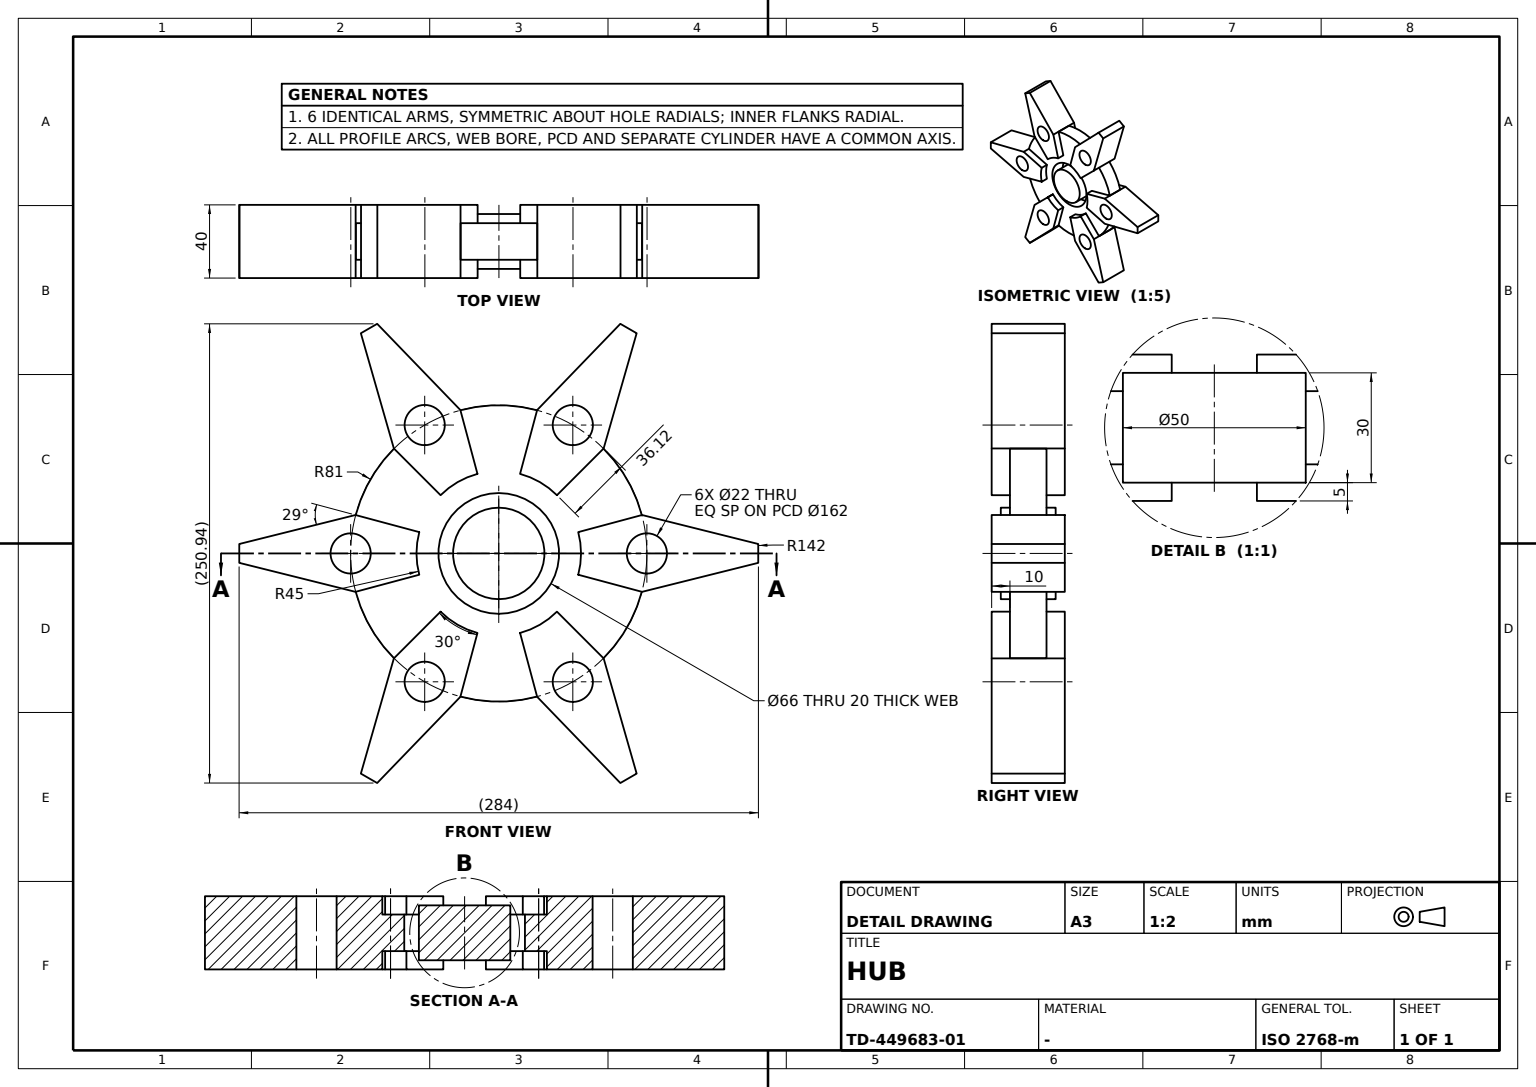
solid
v1 (125.470546,-66.49167,-20)
v2 (125.470546,-66.49167,20)
e1 v1 v2 LINE
v3 (120.318748,-75.414845,20)
e2 v3 v2 CIRCLE(AX(P(0,0,20),D(0,0,1),D(1,0,0)),142)
v4 (120.318748,-75.414845,-20)
e3 v4 v3 LINE
e4 v4 v1 CIRCLE(AX(P(0,0,-20),D(0,0,1),D(1,0,0)),142)
face CYL(AX(P(0,0,0),D(0,0,1),D(0,1,0)),142) [e1 -e2 -e3 e4]
v5 (11.646857,43.466662,20)
v6 (-11.646857,43.466662,20)
e5 v5 v6 CIRCLE(AX(P(0,0,20),D(0,0,1),D(1,0,0)),45)
v7 (-11.646857,43.466662,10)
e6 v7 v6 LINE
v8 (11.646857,43.466662,10)
e7 v8 v7 CIRCLE(AX(P(0,0,10),D(0,0,1),D(1,0,0)),45)
e8 v8 v5 LINE
face CYL(AX(P(0,0,0),D(0,0,1),D(0,1,0)),45) rev [e5 -e6 -e7 e8]
v9 (-31.819805,31.819805,-20)
v10 (-43.466662,11.646857,-20)
e9 v9 v10 CIRCLE(AX(P(0,0,-20),D(0,0,1),D(1,0,0)),45)
v11 (-31.819805,31.819805,-10)
e10 v9 v11 LINE
v12 (-43.466662,11.646857,-10)
e11 v11 v12 CIRCLE(AX(P(0,0,-10),D(0,0,1),D(1,0,0)),45)
e12 v10 v12 LINE
face CYL(AX(P(0,0,0),D(0,0,1),D(0,1,0)),45) rev [-e9 e10 e11 -e12]
v13 (-59.148058,-40.5,-20)
e13 v13 v13 CIRCLE(AX(P(-70.148058,-40.5,-20),D(0,0,1),D(1,0,0)),11)
v14 (-59.148058,-40.5,20)
e14 v14 v14 CIRCLE(AX(P(-70.148058,-40.5,20),D(0,0,1),D(1,0,0)),11)
face CYL(AX(P(-70.148058,-40.5,0),D(0,0,1),D(0,1,0)),11) rev [-e13] [e14]
v15 (-11.646857,-43.466662,20)
v16 (11.646857,-43.466662,20)
e15 v15 v16 CIRCLE(AX(P(0,0,20),D(0,0,1),D(1,0,0)),45)
v17 (11.646857,-43.466662,10)
e16 v17 v16 LINE
v18 (-11.646857,-43.466662,10)
e17 v18 v17 CIRCLE(AX(P(0,0,10),D(0,0,1),D(1,0,0)),45)
e18 v18 v15 LINE
face CYL(AX(P(0,0,0),D(0,0,1),D(0,1,0)),45) rev [e15 -e16 -e17 e18]
v19 (33,0,10)
e19 v19 v19 CIRCLE(AX(P(0,0,10),D(0,0,1),D(1,0,0)),33)
v20 (-20.964343,78.239992,10)
e20 v7 v20 LINE
v21 (-57.275649,57.275649,10)
e21 v20 v21 CIRCLE(AX(P(0,0,10),D(0,0,1),D(1,0,0)),81)
v22 (-31.819805,31.819805,10)
e22 v22 v21 LINE
v23 (-43.466662,11.646857,10)
e23 v22 v23 CIRCLE(AX(P(0,0,10),D(0,0,1),D(1,0,0)),45)
v24 (-78.239992,20.964343,10)
e24 v23 v24 LINE
v25 (-78.239992,-20.964343,10)
e25 v24 v25 CIRCLE(AX(P(0,0,10),D(0,0,1),D(1,0,0)),81)
v26 (-43.466662,-11.646857,10)
e26 v26 v25 LINE
v27 (-31.819805,-31.819805,10)
e27 v26 v27 CIRCLE(AX(P(0,0,10),D(0,0,1),D(1,0,0)),45)
v28 (-57.275649,-57.275649,10)
e28 v27 v28 LINE
v29 (-20.964343,-78.239992,10)
e29 v28 v29 CIRCLE(AX(P(0,0,10),D(0,0,1),D(1,0,0)),81)
e30 v29 v18 LINE
v30 (20.964343,-78.239992,10)
e31 v30 v17 LINE
v31 (57.275649,-57.275649,10)
e32 v30 v31 CIRCLE(AX(P(0,0,10),D(0,0,1),D(1,0,0)),81)
v32 (31.819805,-31.819805,10)
e33 v31 v32 LINE
v33 (43.466662,-11.646857,10)
e34 v32 v33 CIRCLE(AX(P(0,0,10),D(0,0,1),D(1,0,0)),45)
v34 (78.239992,-20.964343,10)
e35 v34 v33 LINE
v35 (78.239992,20.964343,10)
e36 v34 v35 CIRCLE(AX(P(0,0,10),D(0,0,1),D(1,0,0)),81)
v36 (43.466662,11.646857,10)
e37 v35 v36 LINE
v37 (31.819805,31.819805,10)
e38 v36 v37 CIRCLE(AX(P(0,0,10),D(0,0,1),D(1,0,0)),45)
v38 (57.275649,57.275649,10)
e39 v38 v37 LINE
v39 (20.964343,78.239992,10)
e40 v38 v39 CIRCLE(AX(P(0,0,10),D(0,0,1),D(1,0,0)),81)
e41 v8 v39 LINE
face PLANE(AX(P(0,0,10),D(0,0,1),D(0,1,0))) [-e19] [e20 e21 -e22 e23 e24 e25 -e26 e27 e28 e29 e30 e17 -e31 e32 e33 e34 -e35 e36 e37 e38 -e39 e40 -e41 e7]
v40 (-57.275649,-57.275649,-10)
e42 v40 v28 LINE
v41 (-31.819805,-31.819805,20)
e43 v27 v41 LINE
v42 (-57.362403,-57.362403,20)
e44 v41 v42 LINE
v43 (-57.362403,-57.362403,-20)
e45 v43 v42 LINE
v44 (-31.819805,-31.819805,-20)
e46 v44 v43 LINE
v45 (-31.819805,-31.819805,-10)
e47 v44 v45 LINE
e48 v45 v40 LINE
face PLANE(AX(P(-31.819805,-31.819805,0),D(-0.707106781,0.707106781,0),D(-0.707106781,-0.707106781,0))) rev [e42 -e28 e43 e44 -e45 -e46 e47 e48]
v46 (-11.646857,-43.466662,-20)
v47 (-11.646857,-43.466662,-10)
e49 v46 v47 LINE
v48 (11.646857,-43.466662,-10)
e50 v47 v48 CIRCLE(AX(P(0,0,-10),D(0,0,1),D(1,0,0)),45)
v49 (11.646857,-43.466662,-20)
e51 v49 v48 LINE
e52 v46 v49 CIRCLE(AX(P(0,0,-20),D(0,0,1),D(1,0,0)),45)
face CYL(AX(P(0,0,0),D(0,0,1),D(0,1,0)),45) rev [e49 e50 -e51 -e52]
v50 (-57.275649,57.275649,-10)
e53 v11 v50 LINE
v51 (-57.362403,57.362403,-20)
e54 v9 v51 LINE
v52 (-57.362403,57.362403,20)
e55 v51 v52 LINE
v53 (-31.819805,31.819805,20)
e56 v53 v52 LINE
e57 v22 v53 LINE
e58 v50 v21 LINE
face PLANE(AX(P(-31.819805,31.819805,0),D(0.707106781,0.707106781,0),D(-0.707106781,0.707106781,0))) [-e53 -e10 e54 e55 -e56 -e57 e22 -e58]
v54 (-20.964343,78.239992,-10)
e59 v54 v20 LINE
e60 v54 v50 CIRCLE(AX(P(0,0,-10),D(0,0,1),D(1,0,0)),81)
face CYL(AX(P(0,0,0),D(0,0,1),D(0,1,0)),81) [-e21 -e59 e60 e58]
v55 (-59.148058,40.5,20)
e61 v55 v55 CIRCLE(AX(P(-70.148058,40.5,20),D(0,0,1),D(1,0,0)),11)
v56 (-59.148058,40.5,-20)
e62 v56 v56 CIRCLE(AX(P(-70.148058,40.5,-20),D(0,0,1),D(1,0,0)),11)
face CYL(AX(P(-70.148058,40.5,0),D(0,0,1),D(0,1,0)),11) rev [e61] [-e62]
v57 (57.275649,-57.275649,-10)
e63 v57 v31 LINE
v58 (20.964343,-78.239992,-10)
e64 v58 v30 LINE
e65 v58 v57 CIRCLE(AX(P(0,0,-10),D(0,0,1),D(1,0,0)),81)
face CYL(AX(P(0,0,0),D(0,0,1),D(0,1,0)),81) [e63 -e32 -e64 e65]
v59 (20.996097,-78.3585,-20)
v60 (5.151797,-141.906515,-20)
e66 v59 v60 LINE
v61 (-5.151797,-141.906515,-20)
e67 v61 v60 CIRCLE(AX(P(0,0,-20),D(0,0,1),D(1,0,0)),142)
v62 (-20.996097,-78.3585,-20)
e68 v62 v61 LINE
e69 v46 v62 LINE
e70 v49 v59 LINE
v63 (11,-81,-20)
e71 v63 v63 CIRCLE(AX(P(0,-81,-20),D(0,0,1),D(1,0,0)),11)
face PLANE(AX(P(0,0,-20),D(0,0,1),D(0,1,0))) rev [e66 -e67 -e68 -e69 e52 e70] [e71]
v64 (11,81,20)
e72 v64 v64 CIRCLE(AX(P(0,81,20),D(0,0,1),D(1,0,0)),11)
v65 (-20.996097,78.3585,20)
v66 (-5.151797,141.906515,20)
e73 v65 v66 LINE
e74 v6 v65 LINE
v67 (20.996097,78.3585,20)
e75 v5 v67 LINE
v68 (5.151797,141.906515,20)
e76 v67 v68 LINE
e77 v68 v66 CIRCLE(AX(P(0,0,20),D(0,0,1),D(1,0,0)),142)
face PLANE(AX(P(0,0,20),D(0,0,1),D(0,1,0))) [-e72] [-e73 -e74 -e5 e75 e76 e77]
v69 (-78.239992,20.964343,-10)
v70 (-78.239992,-20.964343,-10)
e78 v69 v70 CIRCLE(AX(P(0,0,-10),D(0,0,1),D(1,0,0)),81)
e79 v70 v25 LINE
e80 v69 v24 LINE
face CYL(AX(P(0,0,0),D(0,0,1),D(0,1,0)),81) [e78 e79 -e25 -e80]
v71 (-78.3585,-20.996097,-20)
v72 (-78.3585,-20.996097,20)
e81 v71 v72 LINE
v73 (-125.470546,-66.49167,-20)
e82 v71 v73 LINE
v74 (-125.470546,-66.49167,20)
e83 v73 v74 LINE
e84 v72 v74 LINE
face PLANE(AX(P(-78.3585,-20.996097,0),D(-0.69465837,0.7193398,0),D(-0.7193398,-0.69465837,0))) [-e81 e82 e83 -e84]
v75 (-5.151797,-141.906515,20)
e85 v61 v75 LINE
v76 (-20.996097,-78.3585,20)
e86 v76 v75 LINE
e87 v62 v76 LINE
face PLANE(AX(P(-20.996097,-78.3585,0),D(-0.970295726,-0.241921896,0),D(0.241921896,-0.970295726,0))) [e68 e85 -e86 -e87]
v77 (43.466662,11.646857,-20)
v78 (31.819805,31.819805,-20)
e88 v77 v78 CIRCLE(AX(P(0,0,-20),D(0,0,1),D(1,0,0)),45)
v79 (43.466662,11.646857,-10)
e89 v77 v79 LINE
v80 (31.819805,31.819805,-10)
e90 v79 v80 CIRCLE(AX(P(0,0,-10),D(0,0,1),D(1,0,0)),45)
e91 v78 v80 LINE
face CYL(AX(P(0,0,0),D(0,0,1),D(0,1,0)),45) rev [-e88 e89 e90 -e91]
v81 (-78.3585,20.996097,20)
v82 (-125.470546,66.49167,20)
e92 v81 v82 LINE
v83 (-125.470546,66.49167,-20)
e93 v83 v82 LINE
v84 (-78.3585,20.996097,-20)
e94 v84 v83 LINE
e95 v84 v81 LINE
face PLANE(AX(P(-78.3585,20.996097,0),D(0.69465837,0.7193398,0),D(-0.7193398,0.69465837,0))) rev [e92 -e93 -e94 e95]
v85 (125.470546,66.49167,-20)
v86 (120.318748,75.414845,-20)
e96 v85 v86 CIRCLE(AX(P(0,0,-20),D(0,0,1),D(1,0,0)),142)
v87 (120.318748,75.414845,20)
e97 v86 v87 LINE
v88 (125.470546,66.49167,20)
e98 v88 v87 CIRCLE(AX(P(0,0,20),D(0,0,1),D(1,0,0)),142)
e99 v85 v88 LINE
face CYL(AX(P(0,0,0),D(0,0,1),D(0,1,0)),142) [e96 e97 -e98 -e99]
v89 (5.151797,-141.906515,20)
e100 v75 v89 CIRCLE(AX(P(0,0,20),D(0,0,1),D(1,0,0)),142)
e101 v60 v89 LINE
face CYL(AX(P(0,0,0),D(0,0,1),D(0,1,0)),142) [-e100 -e85 e67 e101]
v90 (-120.318748,75.414845,-20)
v91 (-120.318748,75.414845,20)
e102 v90 v91 LINE
e103 v90 v83 CIRCLE(AX(P(0,0,-20),D(0,0,1),D(1,0,0)),142)
e104 v91 v82 CIRCLE(AX(P(0,0,20),D(0,0,1),D(1,0,0)),142)
face CYL(AX(P(0,0,0),D(0,0,1),D(0,1,0)),142) [-e102 e103 e93 -e104]
v92 (-11.646857,43.466662,-10)
e105 v92 v54 LINE
v93 (11.646857,43.466662,-10)
e106 v93 v92 CIRCLE(AX(P(0,0,-10),D(0,0,1),D(1,0,0)),45)
v94 (20.964343,78.239992,-10)
e107 v93 v94 LINE
v95 (57.275649,57.275649,-10)
e108 v95 v94 CIRCLE(AX(P(0,0,-10),D(0,0,1),D(1,0,0)),81)
e109 v95 v80 LINE
v96 (78.239992,20.964343,-10)
e110 v96 v79 LINE
v97 (78.239992,-20.964343,-10)
e111 v97 v96 CIRCLE(AX(P(0,0,-10),D(0,0,1),D(1,0,0)),81)
v98 (43.466662,-11.646857,-10)
e112 v97 v98 LINE
v99 (31.819805,-31.819805,-10)
e113 v99 v98 CIRCLE(AX(P(0,0,-10),D(0,0,1),D(1,0,0)),45)
e114 v57 v99 LINE
e115 v58 v48 LINE
v100 (-20.964343,-78.239992,-10)
e116 v100 v47 LINE
e117 v40 v100 CIRCLE(AX(P(0,0,-10),D(0,0,1),D(1,0,0)),81)
v101 (-43.466662,-11.646857,-10)
e118 v101 v45 CIRCLE(AX(P(0,0,-10),D(0,0,1),D(1,0,0)),45)
e119 v101 v70 LINE
e120 v12 v69 LINE
v102 (33,0,-10)
e121 v102 v102 CIRCLE(AX(P(0,0,-10),D(0,0,1),D(1,0,0)),33)
face PLANE(AX(P(0,0,-10),D(0,0,1),D(0,1,0))) rev [-e105 -e106 e107 -e108 e109 -e90 -e110 -e111 e112 -e113 -e114 -e65 e115 -e50 -e116 -e117 -e48 -e118 e119 -e78 -e120 -e11 e53 -e60] [e121]
v103 (5.151797,141.906515,-20)
v104 (-5.151797,141.906515,-20)
e122 v103 v104 CIRCLE(AX(P(0,0,-20),D(0,0,1),D(1,0,0)),142)
e123 v104 v66 LINE
e124 v103 v68 LINE
face CYL(AX(P(0,0,0),D(0,0,1),D(0,1,0)),142) [e122 e123 -e77 -e124]
v105 (-43.466662,11.646857,20)
e125 v23 v105 LINE
e126 v105 v81 LINE
e127 v10 v84 LINE
face PLANE(AX(P(-43.466662,11.646857,0),D(0.258819045,0.965925826,0),D(-0.965925826,0.258819045,0))) rev [e125 e126 -e95 -e127 e12 e120 e80 -e24]
v106 (57.362403,57.362403,20)
e128 v106 v87 LINE
v107 (57.362403,57.362403,-20)
e129 v107 v86 LINE
e130 v107 v106 LINE
face PLANE(AX(P(57.362403,57.362403,0),D(0.275637356,-0.961261696,0),D(0.961261696,0.275637356,0))) rev [e128 -e97 -e129 e130]
v108 (20.996097,-78.3585,20)
e131 v16 v108 LINE
e132 v59 v108 LINE
face PLANE(AX(P(-11.646857,43.466662,0),D(0.965925826,0.258819045,0),D(-0.258819045,0.965925826,0))) [-e70 e51 -e115 e64 e31 e16 e131 -e132]
e133 v108 v89 LINE
e134 v15 v76 LINE
v109 (11,-81,20)
e135 v109 v109 CIRCLE(AX(P(0,-81,20),D(0,0,1),D(1,0,0)),11)
face PLANE(AX(P(0,0,20),D(0,0,1),D(0,1,0))) [-e133 -e131 -e15 e134 e86 e100] [-e135]
v110 (78.3585,-20.996097,-20)
e136 v110 v1 LINE
v111 (78.3585,-20.996097,20)
e137 v110 v111 LINE
e138 v111 v2 LINE
face PLANE(AX(P(78.3585,-20.996097,0),D(-0.69465837,-0.7193398,0),D(0.7193398,-0.69465837,0))) rev [-e1 -e136 e137 e138]
v112 (-11.646857,43.466662,-20)
v113 (-20.996097,78.3585,-20)
e139 v112 v113 LINE
e140 v113 v104 LINE
v114 (20.996097,78.3585,-20)
e141 v114 v103 LINE
v115 (11.646857,43.466662,-20)
e142 v115 v114 LINE
e143 v115 v112 CIRCLE(AX(P(0,0,-20),D(0,0,1),D(1,0,0)),45)
v116 (11,81,-20)
e144 v116 v116 CIRCLE(AX(P(0,81,-20),D(0,0,1),D(1,0,0)),11)
face PLANE(AX(P(0,0,-20),D(0,0,1),D(0,1,0))) rev [e139 e140 -e122 -e141 -e142 e143] [e144]
v117 (-43.466662,-11.646857,20)
e145 v117 v72 LINE
e146 v26 v117 LINE
v118 (-43.466662,-11.646857,-20)
e147 v118 v101 LINE
e148 v118 v71 LINE
face PLANE(AX(P(-43.466662,-11.646857,0),D(-0.258819045,0.965925826,0),D(-0.965925826,-0.258819045,0))) [e81 -e145 -e146 e26 -e79 -e119 -e147 e148]
e149 v94 v39 LINE
e150 v115 v93 LINE
e151 v114 v67 LINE
face PLANE(AX(P(11.646857,43.466662,0),D(0.965925826,-0.258819045,0),D(0.258819045,0.965925826,0))) [-e149 -e107 -e150 e142 e151 -e75 -e8 e41]
e152 v100 v29 LINE
face PLANE(AX(P(11.646857,43.466662,0),D(0.965925826,-0.258819045,0),D(0.258819045,0.965925826,0))) rev [e116 -e49 e69 e87 -e134 -e18 -e30 -e152]
v119 (81.148058,40.5,20)
e153 v119 v119 CIRCLE(AX(P(70.148058,40.5,20),D(0,0,1),D(1,0,0)),11)
v120 (31.819805,31.819805,20)
e154 v120 v106 LINE
v121 (43.466662,11.646857,20)
e155 v121 v120 CIRCLE(AX(P(0,0,20),D(0,0,1),D(1,0,0)),45)
v122 (78.3585,20.996097,20)
e156 v121 v122 LINE
e157 v122 v88 LINE
face PLANE(AX(P(0,0,20),D(0,0,1),D(0,1,0))) [-e153] [-e128 -e154 -e155 e156 e157 e98]
e158 v118 v44 CIRCLE(AX(P(0,0,-20),D(0,0,1),D(1,0,0)),45)
v123 (-120.318748,-75.414845,-20)
e159 v43 v123 LINE
e160 v73 v123 CIRCLE(AX(P(0,0,-20),D(0,0,1),D(1,0,0)),142)
face PLANE(AX(P(0,0,-20),D(0,0,1),D(0,1,0))) rev [e13] [-e82 -e148 e158 e46 e159 -e160]
face CYL(AX(P(0,81,0),D(0,0,1),D(0,1,0)),11) rev [-e144] [e72]
e161 v37 v120 LINE
e162 v78 v107 LINE
e163 v95 v38 LINE
face PLANE(AX(P(-31.819805,-31.819805,0),D(-0.707106781,0.707106781,0),D(-0.707106781,-0.707106781,0))) [e39 e161 e154 -e130 -e162 e91 -e109 e163]
v124 (-120.318748,-75.414845,20)
e164 v74 v124 CIRCLE(AX(P(0,0,20),D(0,0,1),D(1,0,0)),142)
e165 v42 v124 LINE
e166 v117 v41 CIRCLE(AX(P(0,0,20),D(0,0,1),D(1,0,0)),45)
face PLANE(AX(P(0,0,20),D(0,0,1),D(0,1,0))) [-e14] [e84 e164 -e165 -e44 -e166 e145]
e167 v36 v121 LINE
face CYL(AX(P(0,0,0),D(0,0,1),D(0,1,0)),45) rev [-e161 -e38 e167 e155]
e168 v113 v65 LINE
e169 v112 v92 LINE
face PLANE(AX(P(-11.646857,43.466662,0),D(0.965925826,0.258819045,0),D(-0.258819045,0.965925826,0))) rev [e6 e74 -e168 -e139 e169 e105 e59 -e20]
face PLANE(AX(P(20.996097,-78.3585,0),D(-0.970295726,0.241921896,0),D(-0.241921896,-0.970295726,0))) rev [e132 e133 -e101 -e66]
face CYL(AX(P(0,0,0),D(0,0,1),D(0,1,0)),81) [-e40 -e163 e108 e149]
face CYL(AX(P(0,0,0),D(0,0,1),D(0,1,0)),81) [e152 -e29 -e42 e117]
v125 (31.819805,-31.819805,20)
v126 (43.466662,-11.646857,20)
e170 v125 v126 CIRCLE(AX(P(0,0,20),D(0,0,1),D(1,0,0)),45)
v127 (57.362403,-57.362403,20)
e171 v125 v127 LINE
e172 v127 v3 LINE
e173 v126 v111 LINE
v128 (81.148058,-40.5,20)
e174 v128 v128 CIRCLE(AX(P(70.148058,-40.5,20),D(0,0,1),D(1,0,0)),11)
face PLANE(AX(P(0,0,20),D(0,0,1),D(0,1,0))) [-e170 e171 e172 e2 -e138 -e173] [-e174]
face CYL(AX(P(0,-81,0),D(0,0,1),D(0,1,0)),11) rev [e135] [-e71]
face PLANE(AX(P(20.996097,78.3585,0),D(0.970295726,0.241921896,0),D(-0.241921896,0.970295726,0))) [e124 -e76 -e151 e141]
v129 (43.466662,-11.646857,-20)
e175 v129 v98 LINE
v130 (31.819805,-31.819805,-20)
e176 v130 v129 CIRCLE(AX(P(0,0,-20),D(0,0,1),D(1,0,0)),45)
e177 v130 v99 LINE
face CYL(AX(P(0,0,0),D(0,0,1),D(0,1,0)),45) rev [-e175 -e176 e177 e113]
e178 v51 v90 LINE
face PLANE(AX(P(0,0,-20),D(0,0,1),D(0,1,0))) rev [e62] [e94 -e103 -e178 -e54 e9 e127]
face CYL(AX(P(0,0,0),D(0,0,1),D(0,1,0)),45) rev [-e143 e150 e106 -e169]
v131 (78.3585,20.996097,-20)
e179 v131 v85 LINE
e180 v131 v122 LINE
face PLANE(AX(P(78.3585,20.996097,0),D(0.69465837,-0.7193398,0),D(0.7193398,0.69465837,0))) [e179 e99 -e157 -e180]
e181 v33 v126 LINE
e182 v32 v125 LINE
face CYL(AX(P(0,0,0),D(0,0,1),D(0,1,0)),45) rev [e170 -e181 -e34 e182]
v132 (57.362403,-57.362403,-20)
e183 v132 v127 LINE
e184 v132 v4 LINE
face PLANE(AX(P(57.362403,-57.362403,0),D(-0.275637356,-0.961261696,0),D(0.961261696,-0.275637356,0))) [-e172 -e183 e184 e3]
v133 (81.148058,40.5,-20)
e185 v133 v133 CIRCLE(AX(P(70.148058,40.5,-20),D(0,0,1),D(1,0,0)),11)
face CYL(AX(P(70.148058,40.5,0),D(0,0,1),D(0,1,0)),11) rev [e153] [-e185]
e186 v77 v131 LINE
face PLANE(AX(P(0,0,-20),D(0,0,1),D(0,1,0))) rev [-e186 e88 e162 e129 -e96 -e179] [e185]
e187 v130 v132 LINE
face PLANE(AX(P(-31.819805,31.819805,0),D(0.707106781,0.707106781,0),D(-0.707106781,0.707106781,0))) rev [e187 e183 -e171 -e182 -e33 -e63 e114 -e177]
v134 (81.148058,-40.5,-20)
e188 v134 v134 CIRCLE(AX(P(70.148058,-40.5,-20),D(0,0,1),D(1,0,0)),11)
face CYL(AX(P(70.148058,-40.5,0),D(0,0,1),D(0,1,0)),11) rev [e174] [-e188]
e189 v123 v124 LINE
face CYL(AX(P(0,0,0),D(0,0,1),D(0,1,0)),142) [e189 -e164 -e83 e160]
face PLANE(AX(P(-57.362403,-57.362403,0),D(-0.275637356,0.961261696,0),D(-0.961261696,-0.275637356,0))) rev [-e159 e45 e165 -e189]
face CYL(AX(P(0,0,0),D(0,0,1),D(0,1,0)),45) rev [-e43 -e27 e146 e166]
e190 v53 v105 CIRCLE(AX(P(0,0,20),D(0,0,1),D(1,0,0)),45)
e191 v52 v91 LINE
face PLANE(AX(P(0,0,20),D(0,0,1),D(0,1,0))) [-e61] [-e126 -e190 e56 e191 e104 -e92]
e192 v129 v110 LINE
e193 v97 v34 LINE
face PLANE(AX(P(-43.466662,11.646857,0),D(0.258819045,0.965925826,0),D(-0.965925826,0.258819045,0))) [e181 e173 -e137 -e192 e175 -e112 e193 e35]
face CYL(AX(P(0,0,0),D(0,0,1),D(0,1,0)),33) rev [-e121] [e19]
e194 v96 v35 LINE
face PLANE(AX(P(-43.466662,-11.646857,0),D(-0.258819045,0.965925826,0),D(-0.965925826,-0.258819045,0))) rev [-e37 -e194 e110 -e89 e186 e180 -e156 -e167]
face CYL(AX(P(0,0,0),D(0,0,1),D(0,1,0)),81) [e111 e194 -e36 -e193]
face PLANE(AX(P(0,0,-20),D(0,0,1),D(0,1,0))) rev [-e187 e176 e192 e136 -e4 -e184] [e188]
face PLANE(AX(P(-57.362403,57.362403,0),D(0.275637356,0.961261696,0),D(-0.961261696,0.275637356,0))) [e178 e102 -e191 -e55]
face PLANE(AX(P(-20.996097,78.3585,0),D(0.970295726,-0.241921896,0),D(0.241921896,0.970295726,0))) rev [-e123 -e140 e168 e73]
face CYL(AX(P(0,0,0),D(0,0,1),D(0,1,0)),45) rev [e118 -e47 -e158 e147]
face CYL(AX(P(0,0,0),D(0,0,1),D(0,1,0)),45) rev [e190 -e125 -e23 e57]
solid
v135 (25,0,-15)
e195 v135 v135 CIRCLE(AX(P(0,0,-15),D(0,0,1),D(1,0,0)),25)
face PLANE(AX(P(0,0,-15),D(0,0,1),D(1,0,0))) rev [-e195]
v136 (25,0,15)
e196 v136 v136 CIRCLE(AX(P(0,0,15),D(0,0,1),D(1,0,0)),25)
face CYL(AX(P(0,0,0),D(0,0,1),D(1,0,0)),25) [-e196] [e195]
face PLANE(AX(P(0,0,15),D(0,0,1),D(1,0,0))) [e196]
